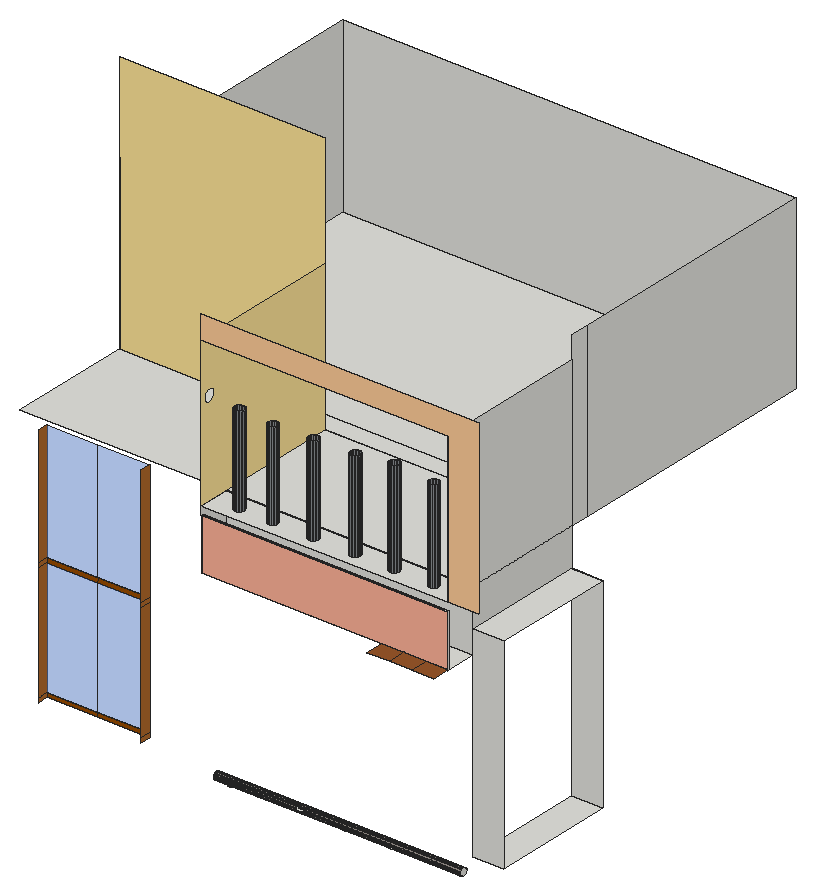
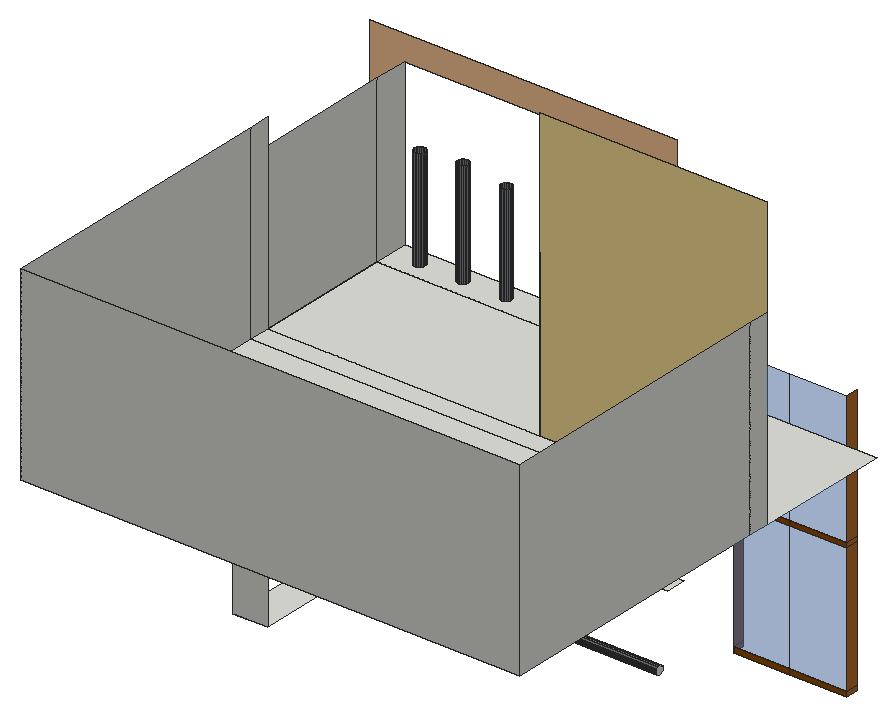
# SketchUp Ruby script. Lengths in inches.
U = 1.inch
M = Sketchup.active_model
def pt(a) = Geom::Point3d.new(a.map { |v| v * U })
def face(e, loops, mat)
  f = e.add_face(loops[0].map { |a| pt(a) })
  loops[1..].each { |l| e.add_face(l.map { |a| pt(a) }).erase! }
  f.material = f.back_material = mat if mat
  f
end
# faces: each face lists its corners as indices into pts; further lists are holes
def faces(e, pts, list, mat = nil) = list.each { |f| face(e, (f[0].is_a?(Array) ? f : [f]).map { |l| l.map { |i| pts[i] } }, mat) }
# xy, xz, yz: faces in a plane at the given z, y or x. An outline is a flat list of corners, or four numbers for a rectangle; further outlines are holes
def ring(l) = l.size == 4 ? [[l[0], l[1]], [l[2], l[1]], [l[2], l[3]], [l[0], l[3]]] : l.each_slice(2).to_a
def flat(e, list, mat, &to3) = list.each { |f| face(e, (f[0].is_a?(Array) ? f : [f]).map { |l| ring(l).map { |u, v| to3.(u, v) } }, mat) }
def xy(e, z, list, mat = nil) = flat(e, list, mat) { |x, y| [x, y, z] }
def xz(e, y, list, mat = nil) = flat(e, list, mat) { |x, z| [x, y, z] }
def yz(e, x, list, mat = nil) = flat(e, list, mat) { |y, z| [x, y, z] }
def lines(e, pts, list) = list.each { |a, b| e.add_line(pt(pts[a]), pt(pts[b])) }
# prism: a flat outline (further loops are holes) pulled along v
def prism(e, loops, v, mat = nil)
  f = face(e, loops, mat); d = Geom::Vector3d.new(v.map { |x| x * U })
  f.pushpull(f.normal.samedirection?(d) ? d.length : -d.length)
end
def box(e, o, s, mat = nil) = prism(e, [[o, [o[0] + s[0], o[1], o[2]], [o[0] + s[0], o[1] + s[1], o[2]], [o[0], o[1] + s[1], o[2]]]], [0, 0, s[2]], mat)
def at(x, y, z, deg = 0) = Geom::Transformation.translation(pt([x, y, z])) * Geom::Transformation.rotation(ORIGIN, Z_AXIS, deg.degrees)
def axes(o, x, y, z) = Geom::Transformation.new([*x, 0, *y, 0, *z, 0, *pt(o).to_a, 1])
def part(name) = M.definitions.add(name)
# library, detail: a bought-in or finely detailed component or shape, given as its bounding box
def library(name, o, s) = part(name).tap { |d| box(d.entities, o, s) }
def detail(e, o, s) = box(e.add_group.entities, o, s)
def put(e, d, t, mat = nil) = e.add_instance(d, t).tap { |i| i.material = mat if mat }
def group(e, t, mat = nil) = e.add_group.tap { |g| g.transformation = t; g.material = mat if mat }.entities
root = M.entities
M.materials.add("[Blacktop Old 01]").color = [132, 136, 139]
M.materials.add("[Color B02]").color = [255, 178, 153]
M.materials.add("[Color C02]").color = [255, 204, 153]
M.materials.add("[Color C07]").color = [153, 76, 0]
M.materials.add("[Color D02]").color = [255, 229, 153]
M.materials.add("[Concrete Scored Jointless]").color = [140, 133, 127]
M.materials.add("[Translucent Glass Blue]").color = [100, 149, 237]
M.materials["[Translucent Glass Blue]"].alpha = 0.5
M.materials.add("[Wood Bamboo]").color = [177, 105, 43]
M.materials.add("[Wood Cherry Original]").color = [152, 86, 42]
xy(root,167.16,[[105.81,78.53,106.15,78.58,106.46,78.71,106.74,78.92,106.95,79.19,107.04,79.42,104.58,79.42,104.67,79.19,104.88,78.92,105.15,78.71,105.47,78.58],[104.58,79.42,107.04,79.42,107.08,79.51,107.12,79.85,107.08,80.1875,106.95,80.5,106.74,80.77,106.46,80.98,106.15,81.11,105.81,81.16,105.47,81.11,105.15,80.98,104.88,80.77,104.67,80.5,104.54,80.1875,104.5,79.85,104.54,79.51]])
xy(root,167.4375,[[114.06,78.53,114.4,78.58,114.71,78.71,114.99,78.92,115.2,79.19,115.27,79.38,112.84,79.38,112.92,79.19,113.13,78.92,113.4,78.71,113.72,78.58],[138.62,78.53,138.96,78.58,139.28,78.71,139.55,78.92,139.76,79.19,139.84,79.38,137.41,79.38,137.48,79.19,137.69,78.92,137.96,78.71,138.28,78.58],[151.93,78.53,152.27,78.58,152.59,78.71,152.86,78.92,153.07,79.19,153.15,79.38,150.72,79.38,150.8,79.19,151.01,78.92,151.28,78.71,151.59,78.58],[112.84,79.38,115.27,79.38,115.33,79.51,115.37,79.85,115.33,80.1875,115.2,80.5,114.99,80.77,114.71,80.98,114.4,81.11,114.06,81.16,113.72,81.11,113.4,80.98,113.13,80.77,112.92,80.5,112.79,80.1875,112.75,79.85,112.79,79.51],[137.41,79.38,139.84,79.38,139.89,79.51,139.93,79.85,139.89,80.1875,139.76,80.5,139.55,80.77,139.28,80.98,138.96,81.11,138.62,81.16,138.28,81.11,137.96,80.98,137.69,80.77,137.48,80.5,137.35,80.1875,137.31,79.85,137.35,79.51],
  [150.72,79.38,153.15,79.38,153.2,79.51,153.25,79.85,153.2,80.1875,153.07,80.5,152.86,80.77,152.59,80.98,152.27,81.11,151.93,81.16,151.59,81.11,151.28,80.98,151.01,80.77,150.8,80.5,150.67,80.1875,150.62,79.85,150.67,79.51]])
xy(root,167.97,[[126,78.53,126.34,78.58,126.65,78.71,126.92,78.92,127.13,79.19,127.26,79.51,127.27,79.52,124.73,79.52,124.73,79.51,124.86,79.19,125.07,78.92,125.34,78.71,125.66,78.58],[124.73,79.52,127.27,79.52,127.31,79.85,127.26,80.1875,127.13,80.5,126.92,80.77,126.65,80.98,126.34,81.11,126,81.16,125.66,81.11,125.34,80.98,125.07,80.77,124.86,80.5,124.73,80.1875,124.68,79.85]])
xy(root,169.8125,[[172.07,83.84,181.07,119.85]])
xy(root,219.0625,[[62.57,119.85,115.13,125.32]])
xy(root,219.5,[[122.02,119.85,166.34,125.32]])
xy(root,222.27,[[100.51,75.28,172.07,83.84]])
xy(root,229.05,[[172.07,83.84,181.07,119.85]])
xy(root,237.59,[[100.51,74.84,172.07,75.28]])
xy(root,240,[[[100.51,74.84,172.07,83.84],[153.24,77.67,152.87,77.72,152.52,77.86,152.22,78.09,151.99,78.39,151.85,78.73,151.8,79.11,151.85,79.48,151.99,79.83,152.22,80.12,152.52,80.35,152.87,80.5,153.24,80.54,153.61,80.5,153.96,80.35,154.26,80.12,154.48,79.83,154.63,79.48,154.68,79.11,154.63,78.73,154.48,78.39,154.26,78.09,153.96,77.86,153.61,77.72],[117.93,77.67,117.56,77.72,117.21,77.86,116.91,78.09,116.68,78.39,116.54,78.73,116.49,79.11,116.54,79.48,116.68,79.83,116.91,80.12,117.21,80.35,117.56,80.5,117.93,80.54,118.3,80.5,118.65,80.35,118.94,80.12,119.17,79.83,119.32,79.48,119.36,79.11,119.32,78.73,119.17,78.39,118.94,78.09,118.65,77.86,118.3,77.72],[141.86,77.67,141.49,77.72,141.15,77.86,140.85,78.09,140.62,78.39,140.48,78.73,140.43,79.11,140.48,79.48,140.62,79.83,140.85,80.12,141.15,80.35,141.49,80.5,141.86,80.54,142.24,80.5,142.58,80.35,142.88,80.12,143.11,79.83,143.25,79.48,143.3,79.11,143.25,78.73,143.11,78.39,142.88,78.09,142.58,77.86,142.24,77.72],[129.74,77.67,129.37,77.72,129.02,77.86,128.72,78.09,128.49,78.39,128.35,78.73,128.3,79.11,128.35,79.48,128.49,79.83,128.72,80.12,129.02,80.35,129.37,80.5,129.74,80.54,130.11,80.5,130.46,80.35,130.76,80.12,130.98,79.83,131.13,79.48,131.18,79.11,131.13,78.73,130.98,78.39,130.76,78.09,130.46,77.86,130.11,77.72],[108.24,77.67,107.87,77.72,107.52,77.86,107.22,78.09,106.99,78.39,106.85,78.73,106.8,79.11,106.85,79.48,106.99,79.83,107.22,80.12,107.52,80.35,107.87,80.5,108.24,80.54,108.61,80.5,108.96,80.35,109.26,80.12,109.48,79.83,109.63,79.48,109.68,79.11,109.63,78.73,109.48,78.39,109.26,78.09,108.96,77.86,108.61,77.72],[164.61,77.67,164.24,77.72,163.9,77.86,163.6,78.09,163.37,78.39,163.23,78.73,163.18,79.11,163.23,79.48,163.37,79.83,163.6,80.12,163.9,80.35,164.24,80.5,164.61,80.54,164.99,80.5,165.33,80.35,165.63,80.12,165.86,79.83,166,79.48,166.05,79.11,166,78.73,165.86,78.39,165.63,78.09,165.33,77.86,164.99,77.72]],[108.24,77.67,107.87,77.72,107.52,77.86,107.22,78.09,106.99,78.39,106.85,78.73,106.8,79.11,106.85,79.48,106.99,79.83,107.22,80.12,107.52,80.35,107.87,80.5,108.24,80.54,108.61,80.5,108.96,80.35,109.26,80.12,109.48,79.83,109.63,79.48,109.68,79.11,109.63,78.73,109.48,78.39,109.26,78.09,108.96,77.86,108.61,77.72],[117.93,77.67,117.56,77.72,117.21,77.86,116.91,78.09,116.68,78.39,116.54,78.73,116.49,79.11,116.54,79.48,116.68,79.83,116.91,80.12,117.21,80.35,117.56,80.5,117.93,80.54,118.3,80.5,118.65,80.35,118.94,80.12,119.17,79.83,119.32,79.48,119.36,79.11,119.32,78.73,119.17,78.39,118.94,78.09,118.65,77.86,118.3,77.72],[129.74,77.67,129.37,77.72,129.02,77.86,128.72,78.09,128.49,78.39,128.35,78.73,128.3,79.11,128.35,79.48,128.49,79.83,128.72,80.12,129.02,80.35,129.37,80.5,129.74,80.54,130.11,80.5,130.46,80.35,130.76,80.12,130.98,79.83,131.13,79.48,131.18,79.11,131.13,78.73,130.98,78.39,130.76,78.09,130.46,77.86,130.11,77.72],[141.86,77.67,141.49,77.72,141.15,77.86,140.85,78.09,140.62,78.39,140.48,78.73,140.43,79.11,140.48,79.48,140.62,79.83,140.85,80.12,141.15,80.35,141.49,80.5,141.86,80.54,142.24,80.5,142.58,80.35,142.88,80.12,143.11,79.83,143.25,79.48,143.3,79.11,143.25,78.73,143.11,78.39,142.88,78.09,142.58,77.86,142.24,77.72],
  [153.24,77.67,152.87,77.72,152.52,77.86,152.22,78.09,151.99,78.39,151.85,78.73,151.8,79.11,151.85,79.48,151.99,79.83,152.22,80.12,152.52,80.35,152.87,80.5,153.24,80.54,153.61,80.5,153.96,80.35,154.26,80.12,154.48,79.83,154.63,79.48,154.68,79.11,154.63,78.73,154.48,78.39,154.26,78.09,153.96,77.86,153.61,77.72],[164.61,77.67,164.24,77.72,163.9,77.86,163.6,78.09,163.37,78.39,163.23,78.73,163.18,79.11,163.23,79.48,163.37,79.83,163.6,80.12,163.9,80.35,164.24,80.5,164.61,80.54,164.99,80.5,165.33,80.35,165.63,80.12,165.86,79.83,166,79.48,166.05,79.11,166,78.73,165.86,78.39,165.63,78.09,165.33,77.86,164.99,77.72],[40.82,83.84,100.51,119.85],[100.51,83.84,172.07,119.85],[40.82,119.85,172.07,125.32],
  [40.82,125.32,172.07,201.03]])
xz(root,74.84,[[172.07,240,181.07,240,181.07,289.8125,100.51,289.8125,100.51,283.17,172.07,283.17]],"[Color C02]")
xz(root,74.84,[[55.76,174.43,70.65,175.68],[70.65,174.43,85.54,175.68],[55.76,209.49,70.65,210.75],[70.65,209.49,85.54,210.75]],"[Color C07]")
xz(root,74.84,[[55.76,175.68,70.65,209.49],[70.65,175.68,85.54,209.49],[55.76,210.75,70.65,245.31],[70.65,210.75,85.54,245.31]],"[Translucent Glass Blue]")
xz(root,75.28,[[100.51,222.27,172.07,237.59]],"[Color B02]")
xz(root,83.84,[[172.07,169.8125,181.07,229.05],[100.51,222.27,172.07,240]])
xz(root,119.85,[[172.07,169.8125,181.07,229.05]])
xz(root,119.85,[[40.82,240,100.51,315.96]],"[Color D02]")
xz(root,201.03,[[40.82,240,172.07,289.8125]])
yz(root,40.82,[[119.85,240,125.32,289.8125],[125.32,240,201.03,289.8125]])
yz(root,55.76,[[71.71,174.43,74.84,175.68],[71.71,175.68,74.84,209.49],[71.71,209.49,74.84,210.75],[71.71,210.75,74.84,245.31]],"[Wood Bamboo]")
yz(root,85.54,[[71.71,174.43,74.84,175.68],[71.71,175.68,74.84,209.49],[71.71,209.49,74.84,210.75],[71.71,210.75,74.84,245.31]],"[Wood Bamboo]")
yz(root,100.51,[[80.44,166.375,80.17,166.41,79.91,166.52,79.69,166.68,79.52,166.9,79.42,167.16,79.38,167.4375,79.42,167.71,79.52,167.97,79.69,168.1875,79.91,168.36,80.17,168.46,80.44,168.5,80.72,168.46,80.97,168.36,81.19,168.1875,81.36,167.97,81.47,167.71,81.51,167.4375,81.47,167.16,81.36,166.9,81.19,166.68,80.97,166.52,80.72,166.41],[75.28,222.27,75.28,237.59,74.84,237.59,74.84,240,83.84,240,83.84,222.27]])
yz(root,100.51,[[[74.84,240,119.85,283.17],[77.85,265.64,77.4,265.7,76.98,265.87,76.62,266.15,76.34,266.51,76.16,266.93,76.1,267.39,76.16,267.84,76.34,268.26,76.62,268.625,76.98,268.9,77.4,269.08,77.85,269.14,78.31,269.08,78.73,268.9,79.09,268.625,79.37,268.26,79.54,267.84,79.6,267.39,79.54,266.93,79.37,266.51,79.09,266.15,78.73,265.87,78.31,265.7]]],"[Color D02]")
yz(root,172.07,[[74.84,222.27,75.28,222.27,74.84,222.28],[75.28,222.27,74.84,222.28,74.84,237.59,75.28,237.59],[83.84,229.05,119.85,240],[74.84,240,83.84,283.17],[83.84,240,119.85,283.17],
  [119.85,240,125.32,289.8125],[125.32,240,201.03,289.8125]])
yz(root,172.2,[[80.44,166.375,80.72,166.41,80.97,166.52,81.19,166.68,81.36,166.9,81.47,167.16,81.51,167.4375,81.47,167.71,81.36,167.97,81.19,168.1875,80.97,168.36,80.72,168.46,80.44,168.5,80.17,168.46,79.91,168.36,79.69,168.1875,79.52,167.97,79.42,167.71,79.38,167.4375,79.42,167.16,79.52,166.9,79.69,166.68,79.91,166.52,80.17,166.41]])
p = [[100.51,79.91,166.52],[100.51,80.17,166.41],[172.2,80.17,166.41],[172.2,79.91,166.52],[100.51,80.44,166.375],[172.2,80.44,166.375],
  [100.51,80.72,166.41],[172.2,80.72,166.41],[100.51,80.97,166.52],[172.2,80.97,166.52],[100.51,79.69,166.68],[172.2,79.69,166.68],
  [100.51,81.19,166.68],[172.2,81.19,166.68],[100.51,79.52,166.9],[172.2,79.52,166.9],[100.51,81.36,166.9],[172.2,81.36,166.9],
  [100.51,79.42,167.16],[172.2,79.42,167.16],[107.04,79.42,167.16],[104.58,79.42,167.16],[100.51,81.47,167.16],[172.2,81.47,167.16],
  [100.51,79.38,167.4375],[172.2,79.38,167.4375],[153.15,79.38,167.4375],[150.72,79.38,167.4375],[139.84,79.38,167.4375],[137.41,79.38,167.4375],
  [115.27,79.38,167.4375],[112.84,79.38,167.4375],[100.51,81.51,167.4375],[172.2,81.51,167.4375],[100.51,79.42,167.71],[172.2,79.42,167.71],
  [100.51,81.47,167.71],[172.2,81.47,167.71],[100.51,79.52,167.97],[172.2,79.52,167.97],[127.27,79.52,167.97],[124.73,79.52,167.97],
  [100.51,81.36,167.97],[172.2,81.36,167.97],[100.51,79.69,168.1875],[172.2,79.69,168.1875],[100.51,81.19,168.1875],[172.2,81.19,168.1875],
  [100.51,79.91,168.36],[172.2,79.91,168.36],[100.51,80.97,168.36],[172.2,80.97,168.36],[100.51,80.17,168.46],[172.2,80.17,168.46],
  [100.51,80.72,168.46],[172.2,80.72,168.46],[100.51,80.44,168.5],[172.2,80.44,168.5],[159.14,75.28,222.27],[152.68,75.28,222.27],
  [152.68,69.9,222.3],[159.14,69.9,222.3],[165.61,75.28,222.27],[165.61,69.9,222.3],[172.07,75.28,222.27],[172.07,69.9,222.3],
  [172.07,74.84,222.28],[107.52,77.86,240],[107.87,77.72,240],[107.87,77.72,266.15],[107.52,77.86,266.15],[108.24,77.67,240],
  [108.24,77.67,266.15],[108.61,77.72,240],[108.61,77.72,266.15],[108.96,77.86,240],[108.96,77.86,266.15],[117.21,77.86,240],
  [117.56,77.72,240],[117.56,77.72,265.4375],[117.21,77.86,265.4375],[117.93,77.67,240],[117.93,77.67,265.4375],[118.3,77.72,240],
  [118.3,77.72,265.4375],[118.65,77.86,240],[118.65,77.86,265.4375],[129.02,77.86,240],[129.37,77.72,240],[129.37,77.72,265.9375],
  [129.02,77.86,265.9375],[129.74,77.67,240],[129.74,77.67,265.9375],[130.11,77.72,240],[130.11,77.72,265.9375],[130.46,77.86,240],
  [130.46,77.86,265.9375],[141.15,77.86,240],[141.49,77.72,240],[141.49,77.72,266.3125],[141.15,77.86,266.3125],[141.86,77.67,240],
  [141.86,77.67,266.3125],[142.24,77.72,240],[142.24,77.72,266.3125],[142.58,77.86,240],[142.58,77.86,266.3125],[152.52,77.86,240],
  [152.87,77.72,240],[152.87,77.72,267.84],[152.52,77.86,267.84],[153.24,77.67,240],[153.24,77.67,267.84],[153.61,77.72,240],
  [153.61,77.72,267.84],[153.96,77.86,240],[153.96,77.86,267.84],[163.9,77.86,240],[164.24,77.72,240],[164.24,77.72,266.75],
  [163.9,77.86,266.75],[164.61,77.67,240],[164.61,77.67,266.75],[164.99,77.72,240],[164.99,77.72,266.75],[165.33,77.86,240],
  [165.33,77.86,266.75],[107.22,78.09,240],[107.22,78.09,266.15],[109.26,78.09,240],[109.26,78.09,266.15],[116.91,78.09,240],
  [116.91,78.09,265.4375],[118.94,78.09,240],[118.94,78.09,265.4375],[128.72,78.09,240],[128.72,78.09,265.9375],[130.76,78.09,240],
  [130.76,78.09,265.9375],[140.85,78.09,240],[140.85,78.09,266.3125],[142.88,78.09,240],[142.88,78.09,266.3125],[152.22,78.09,240],
  [152.22,78.09,267.84],[154.26,78.09,240],[154.26,78.09,267.84],[163.6,78.09,240],[163.6,78.09,266.75],[165.63,78.09,240],
  [165.63,78.09,266.75],[106.99,78.39,240],[106.99,78.39,266.15],[109.48,78.39,240],[109.48,78.39,266.15],[116.68,78.39,240],
  [116.68,78.39,265.4375],[119.17,78.39,240],[119.17,78.39,265.4375],[128.49,78.39,240],[128.49,78.39,265.9375],[130.98,78.39,240],
  [130.98,78.39,265.9375],[140.62,78.39,240],[140.62,78.39,266.3125],[143.11,78.39,240],[143.11,78.39,266.3125],[151.99,78.39,240],
  [151.99,78.39,267.84],[154.48,78.39,240],[154.48,78.39,267.84],[163.37,78.39,240],[163.37,78.39,266.75],[165.86,78.39,240],
  [165.86,78.39,266.75],[106.85,78.73,240],[106.85,78.73,266.15],[109.63,78.73,240],[109.63,78.73,266.15],[116.54,78.73,240],
  [116.54,78.73,265.4375],[119.32,78.73,240],[119.32,78.73,265.4375],[128.35,78.73,240],[128.35,78.73,265.9375],[131.13,78.73,240],
  [131.13,78.73,265.9375],[140.48,78.73,240],[140.48,78.73,266.3125],[143.25,78.73,240],[143.25,78.73,266.3125],[151.85,78.73,240],
  [151.85,78.73,267.84],[154.63,78.73,240],[154.63,78.73,267.84],[163.23,78.73,240],[163.23,78.73,266.75],[166,78.73,240],
  [166,78.73,266.75],[106.8,79.11,240],[106.8,79.09,266.15],[106.8,79.11,266.15],[109.68,79.11,240],[109.68,79.11,266.15],
  [109.68,79.09,266.15],[116.49,79.11,240],[116.49,79.11,265.4375],[119.36,79.11,240],[119.36,79.11,265.4375],[128.3,79.11,240],
  [128.3,79.11,265.9375],[131.18,79.11,240],[131.18,79.11,265.9375],[140.43,79.11,240],[140.43,79.11,266.3125],[143.3,79.11,240],
  [143.3,79.11,266.3125],[151.8,79.11,240],[151.8,79.11,267.84],[154.68,79.11,240],[154.68,79.11,267.84],[163.18,79.11,240],
  [163.18,79.11,266.75],[166.05,79.11,240],[166.05,79.11,266.75],[106.85,79.48,240],[106.85,79.48,266.15],[109.63,79.48,240],
  [109.63,79.48,266.15],[116.54,79.48,240],[116.54,79.48,265.4375],[119.32,79.48,240],[119.32,79.48,265.4375],[128.35,79.48,240],
  [128.35,79.48,265.9375],[131.13,79.48,240],[131.13,79.48,265.9375],[140.48,79.48,240],[140.48,79.48,266.3125],[143.25,79.48,240],
  [143.25,79.48,266.3125],[151.85,79.48,240],[151.85,79.48,267.84],[154.63,79.48,240],[154.63,79.48,267.84],[163.23,79.48,240],
  [163.23,79.48,266.75],[166,79.48,240],[166,79.48,266.75],[106.99,79.83,240],[106.99,79.83,266.15],[109.48,79.83,240],
  [109.48,79.83,266.15],[116.68,79.83,240],[116.68,79.83,265.4375],[119.17,79.83,240],[119.17,79.83,265.4375],[128.49,79.83,240],
  [128.49,79.83,265.9375],[130.98,79.83,240],[130.98,79.83,265.9375],[140.62,79.83,240],[140.62,79.83,266.3125],[143.11,79.83,240],
  [143.11,79.83,266.3125],[151.99,79.83,240],[151.88,79.54,267.84],[151.99,79.83,267.84],[154.48,79.83,240],[154.48,79.83,267.84],
  [154.6,79.54,267.84],[163.37,79.83,240],[163.37,79.83,266.75],[165.86,79.83,240],[165.86,79.83,266.75],[107.22,80.12,240],
  [107.22,80.12,266.15],[109.26,80.12,240],[109.26,80.12,266.15],[116.91,80.12,240],[116.91,80.12,265.4375],[118.94,80.12,240],
  [118.94,80.12,265.4375],[128.72,80.12,240],[128.72,80.12,265.9375],[130.76,80.12,240],[130.76,80.12,265.9375],[140.85,80.12,240],
  [140.85,80.12,266.3125],[142.88,80.12,240],[142.88,80.12,266.3125],[152.22,80.12,240],[152.22,80.12,267.84],[154.26,80.12,240],
  [154.26,80.12,267.84],[163.6,80.12,240],[163.6,80.12,266.75],[165.63,80.12,240],[165.63,80.12,266.75],[107.52,80.35,240],
  [107.52,80.35,266.15],[108.96,80.35,240],[108.96,80.35,266.15],[117.21,80.35,240],[117.21,80.35,265.4375],[118.65,80.35,240],
  [118.65,80.35,265.4375],[129.02,80.35,240],[129.02,80.35,265.9375],[130.46,80.35,240],[130.46,80.35,265.9375],[141.15,80.35,240],
  [141.15,80.35,266.3125],[142.58,80.35,240],[142.58,80.35,266.3125],[152.52,80.35,240],[152.52,80.35,267.84],[153.96,80.35,240],
  [153.96,80.35,267.84],[163.9,80.35,240],[163.9,80.35,266.75],[165.33,80.35,240],[165.33,80.35,266.75],[107.87,80.5,240],
  [107.87,80.5,266.15],[108.61,80.5,240],[108.61,80.5,266.15],[117.56,80.5,240],[117.56,80.5,265.4375],[118.3,80.5,240],
  [118.3,80.5,265.4375],[129.37,80.5,240],[129.37,80.5,265.9375],[130.11,80.5,240],[130.11,80.5,265.9375],[141.49,80.5,240],
  [141.49,80.5,266.3125],[142.24,80.5,240],[142.24,80.5,266.3125],[152.87,80.5,240],[152.87,80.5,267.84],[153.61,80.5,240],
  [153.61,80.5,267.84],[164.24,80.5,240],[164.24,80.5,266.75],[164.99,80.5,240],[164.99,80.5,266.75],[108.24,80.54,240],
  [108.24,80.54,266.15],[117.93,80.54,240],[117.93,80.54,265.4375],[129.74,80.54,240],[129.74,80.54,265.9375],[141.86,80.54,240],
  [141.86,80.54,266.3125],[153.24,80.54,240],[153.24,80.54,267.84],[164.61,80.54,240],[164.61,80.54,266.75]]
faces(root,p,[[0,1,2,3],[1,4,5,2],[4,6,7,5],[6,8,9,7],[10,0,3,11],[8,12,13,9],[14,10,11,15],[12,16,17,13],
  [18,14,15,19,20,21],[16,22,23,17],[24,18,21,20,19,25,26,27,28,29,30,31],[22,32,33,23],[34,24,31,30,29,28,27,26,25,35],[32,36,37,33],[38,34,35,39,40,41],[36,42,43,37],
  [44,38,41,40,39,45],[42,46,47,43],[48,44,45,49],[46,50,51,47],[52,48,49,53],[50,54,55,51],[56,52,53,57],[54,56,57,55]],"[Concrete Scored Jointless]")
faces(root,p,[[58,59,60,61],[62,58,61,63],[64,62,63,65,66]],"[Wood Cherry Original]")
faces(root,p,[[67,68,69,70],[68,71,72,69],[71,73,74,72],[73,75,76,74],[77,78,79,80],[78,81,82,79],[81,83,84,82],[83,85,86,84],
  [87,88,89,90],[88,91,92,89],[91,93,94,92],[93,95,96,94],[97,98,99,100],[98,101,102,99],[101,103,104,102],[103,105,106,104],
  [107,108,109,110],[108,111,112,109],[111,113,114,112],[113,115,116,114],[117,118,119,120],[118,121,122,119],[121,123,124,122],[123,125,126,124],
  [127,67,70,128],[75,129,130,76],[131,77,80,132],[85,133,134,86],[135,87,90,136],[95,137,138,96],[139,97,100,140],[105,141,142,106],
  [143,107,110,144],[115,145,146,116],[147,117,120,148],[125,149,150,126],[151,127,128,152],[129,153,154,130],[155,131,132,156],[133,157,158,134],
  [159,135,136,160],[137,161,162,138],[163,139,140,164],[141,165,166,142],[167,143,144,168],[145,169,170,146],[171,147,148,172],[149,173,174,150],
  [175,151,152,176],[153,177,178,154],[179,155,156,180],[157,181,182,158],[183,159,160,184],[161,185,186,162],[187,163,164,188],[165,189,190,166],
  [191,167,168,192],[169,193,194,170],[195,171,172,196],[173,197,198,174],[199,175,176,200,201],[177,202,203,204,178],[205,179,180,206],[181,207,208,182],
  [209,183,184,210],[185,211,212,186],[213,187,188,214],[189,215,216,190],[217,191,192,218],[193,219,220,194],[221,195,196,222],[197,223,224,198],
  [225,199,201,226],[202,227,228,203],[229,205,206,230],[207,231,232,208],[233,209,210,234],[211,235,236,212],[237,213,214,238],[215,239,240,216],
  [241,217,218,242],[219,243,244,220],[245,221,222,246],[223,247,248,224],[249,225,226,250],[227,251,252,228],[253,229,230,254],[231,255,256,232],
  [257,233,234,258],[235,259,260,236],[261,237,238,262],[239,263,264,240],[265,241,242,266,267],[243,268,269,270,244],[271,245,246,272],[247,273,274,248],
  [275,249,250,276],[251,277,278,252],[279,253,254,280],[255,281,282,256],[283,257,258,284],[259,285,286,260],[287,261,262,288],[263,289,290,264],
  [291,265,267,292],[268,293,294,269],[295,271,272,296],[273,297,298,274],[299,275,276,300],[277,301,302,278],[303,279,280,304],[281,305,306,282],
  [307,283,284,308],[285,309,310,286],[311,287,288,312],[289,313,314,290],[315,291,292,316],[293,317,318,294],[319,295,296,320],[297,321,322,298],
  [323,299,300,324],[301,325,326,302],[327,303,304,328],[305,329,330,306],[331,307,308,332],[309,333,334,310],[335,311,312,336],[313,337,338,314],
  [339,315,316,340],[317,341,342,318],[343,319,320,344],[321,345,346,322],[347,323,324,348],[325,347,348,326],[349,327,328,350],[329,349,350,330],
  [351,331,332,352],[333,351,352,334],[353,335,336,354],[337,353,354,338],[355,339,340,356],[341,355,356,342],[357,343,344,358],[345,357,358,346]],"[Blacktop Old 01]")
